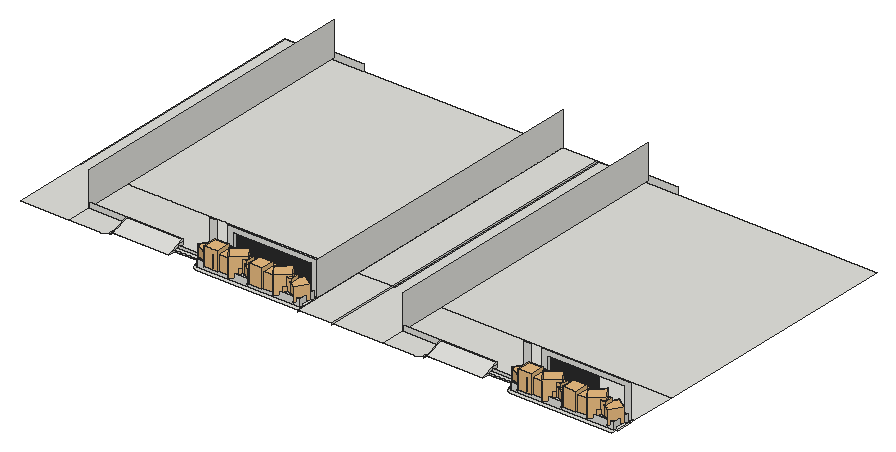
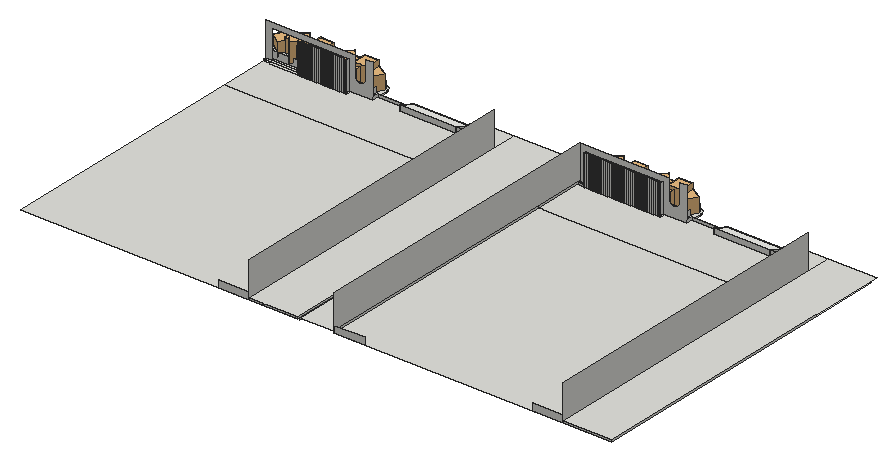
# SketchUp Ruby script. Lengths in inches.
U = 1.inch
M = Sketchup.active_model
def pt(a) = Geom::Point3d.new(a.map { |v| v * U })
def face(e, loops, mat)
  f = e.add_face(loops[0].map { |a| pt(a) })
  loops[1..].each { |l| e.add_face(l.map { |a| pt(a) }).erase! }
  f.material = f.back_material = mat if mat
  f
end
# faces: each face lists its corners as indices into pts; further lists are holes
def faces(e, pts, list, mat = nil) = list.each { |f| face(e, (f[0].is_a?(Array) ? f : [f]).map { |l| l.map { |i| pts[i] } }, mat) }
# xy, xz, yz: faces in a plane at the given z, y or x. An outline is a flat list of corners, or four numbers for a rectangle; further outlines are holes
def ring(l) = l.size == 4 ? [[l[0], l[1]], [l[2], l[1]], [l[2], l[3]], [l[0], l[3]]] : l.each_slice(2).to_a
def flat(e, list, mat, &to3) = list.each { |f| face(e, (f[0].is_a?(Array) ? f : [f]).map { |l| ring(l).map { |u, v| to3.(u, v) } }, mat) }
def xy(e, z, list, mat = nil) = flat(e, list, mat) { |x, y| [x, y, z] }
def xz(e, y, list, mat = nil) = flat(e, list, mat) { |x, z| [x, y, z] }
def yz(e, x, list, mat = nil) = flat(e, list, mat) { |y, z| [x, y, z] }
def lines(e, pts, list) = list.each { |a, b| e.add_line(pt(pts[a]), pt(pts[b])) }
# prism: a flat outline (further loops are holes) pulled along v
def prism(e, loops, v, mat = nil)
  f = face(e, loops, mat); d = Geom::Vector3d.new(v.map { |x| x * U })
  f.pushpull(f.normal.samedirection?(d) ? d.length : -d.length)
end
def box(e, o, s, mat = nil) = prism(e, [[o, [o[0] + s[0], o[1], o[2]], [o[0] + s[0], o[1] + s[1], o[2]], [o[0], o[1] + s[1], o[2]]]], [0, 0, s[2]], mat)
def at(x, y, z, deg = 0) = Geom::Transformation.translation(pt([x, y, z])) * Geom::Transformation.rotation(ORIGIN, Z_AXIS, deg.degrees)
def axes(o, x, y, z) = Geom::Transformation.new([*x, 0, *y, 0, *z, 0, *pt(o).to_a, 1])
def part(name) = M.definitions.add(name)
# library, detail: a bought-in or finely detailed component or shape, given as its bounding box
def library(name, o, s) = part(name).tap { |d| box(d.entities, o, s) }
def detail(e, o, s) = box(e.add_group.entities, o, s)
def put(e, d, t, mat = nil) = e.add_instance(d, t).tap { |i| i.material = mat if mat }
def group(e, t, mat = nil) = e.add_group.tap { |g| g.transformation = t; g.material = mat if mat }.entities
root = M.entities
M.materials.add("Material__1").color = [95, 70, 46]
M.materials.add("[0041_Chocolate]").color = [210, 105, 30]
c1 = library("Areca palm plant",[0,0,0],[49.1,36.6,54.46])
c2 = library("Group\#74",[-84.69,-90.07,-0.36],[176.51,175.13,171.4])
c3 = library("Group20\#1",[-20.81,-17.08,3.79],[39.86,39.43,37.51])
c4 = library("Group38\#2",[14.01,28.44,-23.43],[18.58,18.32,38.89])
c5 = library("Group\#130",[-7.34,-1.2,0],[38.67,35.81,49.04])
c6 = part("Group\#8")
put(c6.entities,c1,axes([-6.2,56.6,6.08],[0.45017,-0.56191,0],[0.66137,0.52986,0],[0,0,0.72]))
put(c6.entities,c1,axes([-6.2,158.41,6.08],[0.45017,-0.56191,0],[0.66137,0.52986,0],[0,0,0.72]))
put(c6.entities,c2,axes([14.93,145.87,6.05],[-0.04961,-0.08593,0],[0.08593,-0.04961,0],[0,0,0.10522]))
put(c6.entities,c2,axes([14.93,193.18,6.05],[-0.04961,-0.08593,0],[0.08593,-0.04961,0],[0,0,0.10522]))
put(c6.entities,c3,axes([18.97,79.98,4.77],[0,0.85,0],[-0.85,0,0],[0,0,0.85]))
put(c6.entities,c2,axes([14.93,173.12,6.05],[-0.04961,-0.08593,0],[0.08593,-0.04961,0],[0,0,0.10522]))
g1 = group(c6.entities,at(0,0,0))
xy(g1,0,[[0,0,6,234.8],[30,0,36,234.8]])
xy(g1,3,[[6,0,30,234.8]])
xy(g1,7,[[6,5,30,229.8]],"Material__1")
xy(g1,15,[[[0,0,36,234.8],[6,5,30,229.8]]])
xz(g1,0,[[0,0,6,0,6,3,30,3,30,0,36,0,36,15,0,15]])
xz(g1,5,[[6,7,30,15]])
xz(g1,229.8,[[6,7,30,15]])
xz(g1,234.8,[[0,0,0,15,36,15,36,0,30,0,30,3,6,3,6,0]])
yz(g1,0,[[0,0,234.8,15]])
yz(g1,6,[[0,0,234.8,3],[5,7,229.8,15]])
yz(g1,30,[[0,0,234.8,3],[5,7,229.8,15]])
yz(g1,36,[[0,0,234.8,15]])
put(c6.entities,c2,axes([17.19,223.04,6.07],[-0.08133,-0.14087,0],[0.14087,-0.08133,0],[0,0,0.1725]))
put(c6.entities,c4,axes([-4.1,-1.15,28.17],[0.8848,0,0],[0,0.94674,0],[0,0,0.85826]))
put(c6.entities,c2,axes([17.19,15.79,6.07],[-0.08133,-0.14087,0],[0.14087,-0.08133,0],[0,0,0.1725]))
put(c6.entities,c2,axes([14.93,91.37,6.05],[-0.04961,-0.08593,0],[0.08593,-0.04961,0],[0,0,0.10522]))
put(c6.entities,c3,axes([18.97,181.79,4.77],[0,0.85,0],[-0.85,0,0],[0,0,0.85]))
put(c6.entities,c2,axes([14.93,44.05,6.05],[-0.04961,-0.08593,0],[0.08593,-0.04961,0],[0,0,0.10522]))
put(c6.entities,c5,axes([24.9375,191.72,8],[0,0.79,0],[-0.79,0,0],[0,0,0.79]))
put(c6.entities,c2,axes([17.19,121.23,6.07],[-0.08133,-0.14087,0],[0.14087,-0.08133,0],[0,0,0.1725]))
put(c6.entities,c4,axes([-4.1,100.66,28.17],[0.8848,0,0],[0,0.94674,0],[0,0,0.85826]))
put(c6.entities,c5,axes([24.9375,89.91,8],[0,0.79,0],[-0.79,0,0],[0,0,0.79]))
put(c6.entities,c2,axes([14.93,71.3,6.05],[-0.04961,-0.08593,0],[0.08593,-0.04961,0],[0,0,0.10522]))
xy(root,-8,[[762.73,853.22,811.8125,853.22,811.8125,894.77,813.4375,894.77,813.4375,895.77,814.1875,895.77,814.1875,894.77,817.4375,894.77,817.4375,895.77,818.1875,895.77,818.1875,894.77,821.4375,894.77,821.4375,895.77,822.1875,895.77,822.1875,894.77,825.4375,894.77,825.4375,895.77,826.1875,895.77,826.1875,894.77,829.4375,894.77,829.4375,895.77,830.1875,895.77,830.1875,894.77,833.4375,894.77,833.4375,895.77,834.1875,895.77,834.1875,894.77,837.4375,894.77,837.4375,895.77,838.1875,895.77,838.1875,894.77,841.4375,894.77,841.4375,895.77,842.1875,895.77,842.1875,894.77,845.4375,894.77,845.4375,895.77,846.1875,895.77,846.1875,894.77,849.4375,894.77,849.4375,895.77,850.1875,895.77,850.1875,894.77,853.4375,894.77,853.4375,895.77,854.1875,895.77,854.1875,894.77,857.4375,894.77,857.4375,895.77,858.1875,895.77,858.1875,894.77,861.4375,894.77,861.4375,895.77,862.1875,895.77,862.1875,894.77,865.4375,894.77,865.4375,895.77,866.1875,895.77,866.1875,894.77,869.4375,894.77,869.4375,895.77,870.1875,895.77,870.1875,894.77,873.4375,894.77,873.4375,895.77,874.1875,895.77,874.1875,894.77,877.4375,894.77,877.4375,895.77,878.1875,895.77,878.1875,894.77,881.4375,894.77,881.4375,895.77,882.1875,895.77,882.1875,894.77,885.4375,894.77,885.4375,895.77,886.1875,895.77,886.1875,894.77,889.4375,894.77,889.4375,895.77,890.1875,895.77,890.1875,894.77,893.4375,894.77,893.4375,895.77,894.1875,895.77,894.1875,894.77,897.4375,894.77,897.4375,895.77,898.1875,895.77,898.1875,894.77,901.4375,894.77,901.4375,895.77,902.1875,895.77,902.1875,894.77,905.4375,894.77,905.4375,895.77,906.1875,895.77,906.1875,894.77,909.4375,894.77,909.4375,895.77,910.1875,895.77,910.1875,894.77,913.4375,894.77,913.4375,895.77,914.1875,895.77,914.1875,894.77,917.4375,894.77,917.4375,895.77,918.1875,895.77,918.1875,894.77,921.4375,894.77,921.4375,895.77,922.1875,895.77,922.1875,894.77,925.4375,894.77,925.4375,895.77,926.1875,895.77,926.1875,894.77,929.4375,894.77,929.4375,895.77,930.1875,895.77,930.1875,894.77,933.4375,894.77,933.4375,895.77,934.1875,895.77,934.1875,894.77,937.4375,894.77,937.4375,895.77,938.1875,895.77,938.1875,894.77,941.4375,894.77,941.4375,895.77,942.1875,895.77,942.1875,894.77,945.4375,894.77,945.4375,895.77,946.1875,895.77,946.1875,894.77,949.4375,894.77,949.4375,895.77,950.1875,895.77,950.1875,894.77,953.4375,894.77,953.4375,895.77,954.1875,895.77,954.1875,894.77,957.4375,894.77,957.4375,895.77,958.1875,895.77,958.1875,894.77,961.4375,894.77,961.4375,895.77,962.1875,895.77,962.1875,894.77,965.4375,894.77,965.4375,895.77,966.1875,895.77,966.1875,894.77,969.4375,894.77,969.4375,895.77,970.1875,895.77,970.1875,894.77,986.33,894.77,986.33,996.48,407.52,996.48,407.52,853.41,705.71,853.41,705.71,868.96,762.73,868.96],[811.8125,853.22,811.8125,894.77,973.4375,894.77,973.4375,889.52,986.33,889.52,986.33,853.22],[1418.23,853.22,1467.3125,853.22,1467.3125,894.77,1468.9375,894.77,1468.9375,895.77,1469.6875,895.77,1469.6875,894.77,1472.9375,894.77,1472.9375,895.77,1473.6875,895.77,1473.6875,894.77,1476.9375,894.77,1476.9375,895.77,1477.6875,895.77,1477.6875,894.77,1480.9375,894.77,1480.9375,895.77,1481.6875,895.77,1481.6875,894.77,1484.9375,894.77,1484.9375,895.77,1485.6875,895.77,1485.6875,894.77,1488.9375,894.77,1488.9375,895.77,1489.6875,895.77,1489.6875,894.77,1492.9375,894.77,1492.9375,895.77,1493.6875,895.77,1493.6875,894.77,1496.9375,894.77,1496.9375,895.77,1497.6875,895.77,1497.6875,894.77,1500.9375,894.77,1500.9375,895.77,1501.6875,895.77,1501.6875,894.77,1504.9375,894.77,1504.9375,895.77,1505.6875,895.77,1505.6875,894.77,1508.9375,894.77,1508.9375,895.77,1509.6875,895.77,1509.6875,894.77,1512.9375,894.77,1512.9375,895.77,1513.6875,895.77,1513.6875,894.77,1516.9375,894.77,1516.9375,895.77,1517.6875,895.77,1517.6875,894.77,1520.9375,894.77,1520.9375,895.77,1521.6875,895.77,1521.6875,894.77,1524.9375,894.77,1524.9375,895.77,1525.6875,895.77,1525.6875,894.77,1528.9375,894.77,1528.9375,895.77,1529.6875,895.77,1529.6875,894.77,1532.9375,894.77,1532.9375,895.77,1533.6875,895.77,1533.6875,894.77,1536.9375,894.77,1536.9375,895.77,1537.6875,895.77,1537.6875,894.77,1540.9375,894.77,1540.9375,895.77,1541.6875,895.77,1541.6875,894.77,1544.9375,894.77,1544.9375,895.77,1545.6875,895.77,1545.6875,894.77,1548.9375,894.77,1548.9375,895.77,1549.6875,895.77,1549.6875,894.77,1552.9375,894.77,1552.9375,895.77,1553.6875,895.77,1553.6875,894.77,1556.9375,894.77,1556.9375,895.77,1557.6875,895.77,1557.6875,894.77,1560.9375,894.77,1560.9375,895.77,1561.6875,895.77,1561.6875,894.77,1564.9375,894.77,1564.9375,895.77,1565.6875,895.77,1565.6875,894.77,1568.9375,894.77,1568.9375,895.77,1569.6875,895.77,1569.6875,894.77,1572.9375,894.77,1572.9375,895.77,1573.6875,895.77,1573.6875,894.77,1576.9375,894.77,1576.9375,895.77,1577.6875,895.77,1577.6875,894.77,1580.9375,894.77,1580.9375,895.77,1581.6875,895.77,1581.6875,894.77,1584.9375,894.77,1584.9375,895.77,1585.6875,895.77,1585.6875,894.77,1588.9375,894.77,1588.9375,895.77,1589.6875,895.77,1589.6875,894.77,1592.9375,894.77,1592.9375,895.77,1593.6875,895.77,1593.6875,894.77,1596.9375,894.77,1596.9375,895.77,1597.6875,895.77,1597.6875,894.77,1600.9375,894.77,1600.9375,895.77,1601.6875,895.77,1601.6875,894.77,1604.9375,894.77,1604.9375,895.77,1605.6875,895.77,1605.6875,894.77,1608.9375,894.77,1608.9375,895.77,1609.6875,895.77,1609.6875,894.77,1612.9375,894.77,1612.9375,895.77,1613.6875,895.77,1613.6875,894.77,1616.9375,894.77,1616.9375,895.77,1617.6875,895.77,1617.6875,894.77,1620.9375,894.77,1620.9375,895.77,1621.6875,895.77,1621.6875,894.77,1624.9375,894.77,1624.9375,895.77,1625.6875,895.77,1625.6875,894.77,1641.83,894.77,1641.83,996.48,1063.02,996.48,1063.02,853.41,1361.21,853.41,1361.21,868.96,1418.23,868.96],[1467.3125,853.22,1467.3125,894.77,1628.9375,894.77,1628.9375,889.52,1641.83,889.52,1641.83,853.22],[973.4375,889.52,986.33,894.77],
  [407.52,996.48,986.33,1529.04],[1063.02,996.48,1641.83,1529.04]])
xy(root,-4.67,[[407.52,838.14,508.71,1529.04],[508.71,838.14,573,838.14,575,838.27,576.96,838.66,578.85,839.31,580.64,840.19,582.3,841.3,583.8,842.62,585.12,844.12,586.23,845.78,587.11,847.57,587.75,849.46,588.14,851.42,588.27,853.41,588.27,889.52,508.71,889.52],[777.8125,838.14,986.33,838.14,986.33,889.52,762.73,889.52,762.73,853.22,762.86,851.26,763.24,849.32,763.88,847.45,764.75,845.68,765.85,844.04,767.15,842.5625,768.63,841.26,770.27,840.16,772.04,839.29,773.91,838.66,775.84,838.27],[986.33,838.14,1058.02,996.48],[1063.02,838.14,1164.21,1529.04],
  [1164.21,838.14,1228.5,838.14,1230.5,838.27,1232.46,838.66,1234.35,839.31,1236.14,840.19,1237.8,841.3,1239.3,842.62,1240.62,844.12,1241.73,845.78,1242.61,847.57,1243.25,849.46,1243.64,851.42,1243.77,853.41,1243.77,889.52,1164.21,889.52],[1433.3125,838.14,1641.83,838.14,1641.83,889.52,1418.23,889.52,1418.23,853.22,1418.36,851.26,1418.74,849.32,1419.38,847.45,1420.25,845.68,1421.35,844.04,1422.65,842.5625,1424.13,841.26,1425.77,840.16,1427.54,839.29,1429.41,838.66,1431.34,838.27],[705.71,868.96,762.73,876.83],[1361.21,868.96,1418.23,876.83],[811.8125,889.52,986.33,894.77],
  [1467.3125,889.52,1641.83,894.77],[986.33,996.48,1058.02,1529.04]])
xz(root,868.96,[[705.71,-8,762.73,-4.67],[1361.21,-8,1418.23,-4.67]])
xz(root,876.83,[[705.71,-4.67,762.73,0.73],[1361.21,-4.67,1418.23,0.73]])
xz(root,889.52,[[973.4375,-8,986.33,-4.67],[508.71,-4.67,588.27,6.125],[588.27,-4.67,705.71,6.125],[762.73,-4.67,811.8125,-4.67,811.8125,55.1875,973.4375,55.1875,973.4375,-4.67,986.33,-4.67,986.33,66.125,800.41,66.125,800.41,26.79,799.52,24.11,798.06,21.71,796.09,19.69,793.71,18.17,791.05,17.23,788.25,16.91,785.45,17.23,782.8,18.17,780.42,19.69,778.45,21.71,776.98,24.11,776.1,26.79,776.1,66.125,762.97,66.125,762.97,6.125,762.73,6.125],[1164.21,-4.67,1243.77,6.125],
  [1243.77,-4.67,1361.21,6.125],[1418.23,-4.67,1467.3125,-4.67,1467.3125,55.1875,1628.9375,55.1875,1628.9375,-4.67,1641.83,-4.67,1641.83,66.125,1455.91,66.125,1455.91,26.79,1455.02,24.11,1453.56,21.71,1451.59,19.69,1449.21,18.17,1446.55,17.23,1443.75,16.91,1440.95,17.23,1438.3,18.17,1435.92,19.69,1433.95,21.71,1432.48,24.11,1431.6,26.79,1431.6,66.125,1418.47,66.125,1418.47,6.125,1418.23,6.125]])
xz(root,894.77,[[811.8125,-8,813.4375,-4.67],[813.4375,-8,814.1875,-4.67],[814.1875,-8,817.4375,-4.67],[817.4375,-8,818.1875,-4.67],[818.1875,-8,821.4375,-4.67],
  [821.4375,-8,822.1875,-4.67],[822.1875,-8,825.4375,-4.67],[825.4375,-8,826.1875,-4.67],[826.1875,-8,829.4375,-4.67],[829.4375,-8,830.1875,-4.67],
  [830.1875,-8,833.4375,-4.67],[833.4375,-8,834.1875,-4.67],[834.1875,-8,837.4375,-4.67],[837.4375,-8,838.1875,-4.67],[838.1875,-8,841.4375,-4.67],
  [841.4375,-8,842.1875,-4.67],[842.1875,-8,845.4375,-4.67],[845.4375,-8,846.1875,-4.67],[846.1875,-8,849.4375,-4.67],[849.4375,-8,850.1875,-4.67],
  [850.1875,-8,853.4375,-4.67],[853.4375,-8,854.1875,-4.67],[854.1875,-8,857.4375,-4.67],[857.4375,-8,858.1875,-4.67],[858.1875,-8,861.4375,-4.67],
  [861.4375,-8,862.1875,-4.67],[862.1875,-8,865.4375,-4.67],[865.4375,-8,866.1875,-4.67],[866.1875,-8,869.4375,-4.67],[869.4375,-8,870.1875,-4.67],
  [870.1875,-8,873.4375,-4.67],[873.4375,-8,874.1875,-4.67],[874.1875,-8,877.4375,-4.67],[877.4375,-8,878.1875,-4.67],[878.1875,-8,881.4375,-4.67],
  [881.4375,-8,882.1875,-4.67],[882.1875,-8,885.4375,-4.67],[885.4375,-8,886.1875,-4.67],[886.1875,-8,889.4375,-4.67],[889.4375,-8,890.1875,-4.67],
  [890.1875,-8,893.4375,-4.67],[893.4375,-8,894.1875,-4.67],[894.1875,-8,897.4375,-4.67],[897.4375,-8,898.1875,-4.67],[898.1875,-8,901.4375,-4.67],
  [901.4375,-8,902.1875,-4.67],[902.1875,-8,905.4375,-4.67],[905.4375,-8,906.1875,-4.67],[906.1875,-8,909.4375,-4.67],[909.4375,-8,910.1875,-4.67],
  [910.1875,-8,913.4375,-4.67],[913.4375,-8,914.1875,-4.67],[914.1875,-8,917.4375,-4.67],[917.4375,-8,918.1875,-4.67],[918.1875,-8,921.4375,-4.67],
  [921.4375,-8,922.1875,-4.67],[922.1875,-8,925.4375,-4.67],[925.4375,-8,926.1875,-4.67],[926.1875,-8,929.4375,-4.67],[929.4375,-8,930.1875,-4.67],
  [930.1875,-8,933.4375,-4.67],[933.4375,-8,934.1875,-4.67],[934.1875,-8,937.4375,-4.67],[937.4375,-8,938.1875,-4.67],[938.1875,-8,941.4375,-4.67],
  [941.4375,-8,942.1875,-4.67],[942.1875,-8,945.4375,-4.67],[945.4375,-8,946.1875,-4.67],[946.1875,-8,949.4375,-4.67],[949.4375,-8,950.1875,-4.67],
  [950.1875,-8,953.4375,-4.67],[953.4375,-8,954.1875,-4.67],[954.1875,-8,957.4375,-4.67],[957.4375,-8,958.1875,-4.67],[958.1875,-8,961.4375,-4.67],
  [961.4375,-8,962.1875,-4.67],[962.1875,-8,965.4375,-4.67],[965.4375,-8,966.1875,-4.67],[966.1875,-8,969.4375,-4.67],[969.4375,-8,970.1875,-4.67],
  [970.1875,-8,973.4375,-4.67],[973.4375,-8,986.33,-4.67],[1467.3125,-8,1468.9375,-4.67],[1468.9375,-8,1469.6875,-4.67],[1469.6875,-8,1472.9375,-4.67],
  [1472.9375,-8,1473.6875,-4.67],[1473.6875,-8,1476.9375,-4.67],[1476.9375,-8,1477.6875,-4.67],[1477.6875,-8,1480.9375,-4.67],[1480.9375,-8,1481.6875,-4.67],
  [1481.6875,-8,1484.9375,-4.67],[1484.9375,-8,1485.6875,-4.67],[1485.6875,-8,1488.9375,-4.67],[1488.9375,-8,1489.6875,-4.67],[1489.6875,-8,1492.9375,-4.67],
  [1492.9375,-8,1493.6875,-4.67],[1493.6875,-8,1496.9375,-4.67],[1496.9375,-8,1497.6875,-4.67],[1497.6875,-8,1500.9375,-4.67],[1500.9375,-8,1501.6875,-4.67],
  [1501.6875,-8,1504.9375,-4.67],[1504.9375,-8,1505.6875,-4.67],[1505.6875,-8,1508.9375,-4.67],[1508.9375,-8,1509.6875,-4.67],[1509.6875,-8,1512.9375,-4.67],
  [1512.9375,-8,1513.6875,-4.67],[1513.6875,-8,1516.9375,-4.67],[1516.9375,-8,1517.6875,-4.67],[1517.6875,-8,1520.9375,-4.67],[1520.9375,-8,1521.6875,-4.67],
  [1521.6875,-8,1524.9375,-4.67],[1524.9375,-8,1525.6875,-4.67],[1525.6875,-8,1528.9375,-4.67],[1528.9375,-8,1529.6875,-4.67],[1529.6875,-8,1532.9375,-4.67],
  [1532.9375,-8,1533.6875,-4.67],[1533.6875,-8,1536.9375,-4.67],[1536.9375,-8,1537.6875,-4.67],[1537.6875,-8,1540.9375,-4.67],[1540.9375,-8,1541.6875,-4.67],
  [1541.6875,-8,1544.9375,-4.67],[1544.9375,-8,1545.6875,-4.67],[1545.6875,-8,1548.9375,-4.67],[1548.9375,-8,1549.6875,-4.67],[1549.6875,-8,1552.9375,-4.67],
  [1552.9375,-8,1553.6875,-4.67],[1553.6875,-8,1556.9375,-4.67],[1556.9375,-8,1557.6875,-4.67],[1557.6875,-8,1560.9375,-4.67],[1560.9375,-8,1561.6875,-4.67],
  [1561.6875,-8,1564.9375,-4.67],[1564.9375,-8,1565.6875,-4.67],[1565.6875,-8,1568.9375,-4.67],[1568.9375,-8,1569.6875,-4.67]])
xz(root,894.77,[[811.8125,-4.67,813.4375,55.1875],[814.1875,-4.67,817.4375,55.1875],[818.1875,-4.67,821.4375,55.1875],[822.1875,-4.67,825.4375,55.1875],[826.1875,-4.67,829.4375,55.1875],
  [830.1875,-4.67,833.4375,55.1875],[834.1875,-4.67,837.4375,55.1875],[838.1875,-4.67,841.4375,55.1875],[842.1875,-4.67,845.4375,55.1875],[846.1875,-4.67,849.4375,55.1875],
  [850.1875,-4.67,853.4375,55.1875],[854.1875,-4.67,857.4375,55.1875],[858.1875,-4.67,861.4375,55.1875],[862.1875,-4.67,865.4375,55.1875],[866.1875,-4.67,869.4375,55.1875],
  [870.1875,-4.67,873.4375,55.1875],[874.1875,-4.67,877.4375,55.1875],[878.1875,-4.67,881.4375,55.1875],[882.1875,-4.67,885.4375,55.1875],[886.1875,-4.67,889.4375,55.1875],
  [890.1875,-4.67,893.4375,55.1875],[894.1875,-4.67,897.4375,55.1875],[898.1875,-4.67,901.4375,55.1875],[902.1875,-4.67,905.4375,55.1875],[906.1875,-4.67,909.4375,55.1875],
  [910.1875,-4.67,913.4375,55.1875],[914.1875,-4.67,917.4375,55.1875],[918.1875,-4.67,921.4375,55.1875],[922.1875,-4.67,925.4375,55.1875],[926.1875,-4.67,929.4375,55.1875],
  [930.1875,-4.67,933.4375,55.1875],[934.1875,-4.67,937.4375,55.1875],[938.1875,-4.67,941.4375,55.1875],[942.1875,-4.67,945.4375,55.1875],[946.1875,-4.67,949.4375,55.1875],
  [950.1875,-4.67,953.4375,55.1875],[954.1875,-4.67,957.4375,55.1875],[958.1875,-4.67,961.4375,55.1875],[962.1875,-4.67,965.4375,55.1875],[966.1875,-4.67,969.4375,55.1875],
  [970.1875,-4.67,973.4375,55.1875],[1467.3125,-4.67,1468.9375,55.1875],[1469.6875,-4.67,1472.9375,55.1875],[1473.6875,-4.67,1476.9375,55.1875],[1477.6875,-4.67,1480.9375,55.1875],
  [1481.6875,-4.67,1484.9375,55.1875],[1485.6875,-4.67,1488.9375,55.1875],[1489.6875,-4.67,1492.9375,55.1875],[1493.6875,-4.67,1496.9375,55.1875],[1497.6875,-4.67,1500.9375,55.1875],
  [1501.6875,-4.67,1504.9375,55.1875],[1505.6875,-4.67,1508.9375,55.1875],[1509.6875,-4.67,1512.9375,55.1875],[1513.6875,-4.67,1516.9375,55.1875],[1517.6875,-4.67,1520.9375,55.1875],
  [1521.6875,-4.67,1524.9375,55.1875],[1525.6875,-4.67,1528.9375,55.1875],[1529.6875,-4.67,1532.9375,55.1875],[1533.6875,-4.67,1536.9375,55.1875],[1537.6875,-4.67,1540.9375,55.1875],
  [1541.6875,-4.67,1544.9375,55.1875],[1545.6875,-4.67,1548.9375,55.1875],[1549.6875,-4.67,1552.9375,55.1875],[1553.6875,-4.67,1556.9375,55.1875],[1557.6875,-4.67,1560.9375,55.1875],
  [1561.6875,-4.67,1564.9375,55.1875],[1565.6875,-4.67,1568.9375,55.1875]],"[0041_Chocolate]")
xz(root,895.77,[[813.4375,-8,814.1875,55.1875],[817.4375,-8,818.1875,55.1875],[821.4375,-8,822.1875,55.1875],[825.4375,-8,826.1875,55.1875],[829.4375,-8,830.1875,55.1875],
  [833.4375,-8,834.1875,55.1875],[837.4375,-8,838.1875,55.1875],[841.4375,-8,842.1875,55.1875],[845.4375,-8,846.1875,55.1875],[849.4375,-8,850.1875,55.1875],
  [853.4375,-8,854.1875,55.1875],[857.4375,-8,858.1875,55.1875],[861.4375,-8,862.1875,55.1875],[865.4375,-8,866.1875,55.1875],[869.4375,-8,870.1875,55.1875],
  [873.4375,-8,874.1875,55.1875],[877.4375,-8,878.1875,55.1875],[881.4375,-8,882.1875,55.1875],[885.4375,-8,886.1875,55.1875],[889.4375,-8,890.1875,55.1875],
  [893.4375,-8,894.1875,55.1875],[897.4375,-8,898.1875,55.1875],[901.4375,-8,902.1875,55.1875],[905.4375,-8,906.1875,55.1875],[909.4375,-8,910.1875,55.1875],
  [913.4375,-8,914.1875,55.1875],[917.4375,-8,918.1875,55.1875],[921.4375,-8,922.1875,55.1875],[925.4375,-8,926.1875,55.1875],[929.4375,-8,930.1875,55.1875],
  [933.4375,-8,934.1875,55.1875],[937.4375,-8,938.1875,55.1875],[941.4375,-8,942.1875,55.1875],[945.4375,-8,946.1875,55.1875],[949.4375,-8,950.1875,55.1875],
  [953.4375,-8,954.1875,55.1875],[957.4375,-8,958.1875,55.1875],[961.4375,-8,962.1875,55.1875],[965.4375,-8,966.1875,55.1875],[969.4375,-8,970.1875,55.1875],
  [1468.9375,-8,1469.6875,55.1875],[1472.9375,-8,1473.6875,55.1875],[1476.9375,-8,1477.6875,55.1875],[1480.9375,-8,1481.6875,55.1875],[1484.9375,-8,1485.6875,55.1875],
  [1488.9375,-8,1489.6875,55.1875],[1492.9375,-8,1493.6875,55.1875],[1496.9375,-8,1497.6875,55.1875],[1500.9375,-8,1501.6875,55.1875],[1504.9375,-8,1505.6875,55.1875],
  [1508.9375,-8,1509.6875,55.1875],[1512.9375,-8,1513.6875,55.1875],[1516.9375,-8,1517.6875,55.1875],[1520.9375,-8,1521.6875,55.1875],[1524.9375,-8,1525.6875,55.1875],
  [1528.9375,-8,1529.6875,55.1875],[1532.9375,-8,1533.6875,55.1875],[1536.9375,-8,1537.6875,55.1875],[1540.9375,-8,1541.6875,55.1875],[1544.9375,-8,1545.6875,55.1875],
  [1548.9375,-8,1549.6875,55.1875],[1552.9375,-8,1553.6875,55.1875],[1556.9375,-8,1557.6875,55.1875],[1560.9375,-8,1561.6875,55.1875],[1564.9375,-8,1565.6875,55.1875],
  [1568.9375,-8,1569.6875,55.1875]])
xz(root,1529.04,[[407.52,-8,407.52,-4.67,508.71,-4.67,508.71,6.125,572.21,6.125,572.21,-8],[922.83,-8,986.33,6.125],[1063.02,-8,1063.02,-4.67,1164.21,-4.67,1164.21,6.125,1227.71,6.125,1227.71,-8]])
yz(root,407.52,[[996.48,-8,1529.04,-4.67]])
yz(root,508.71,[[889.52,-4.67,1529.04,66.125]])
yz(root,588.27,[[853.41,-8,861.93,-4.67,853.41,-4.67],[861.93,-4.67,889.52,6.125,889.52,-4.67]])
yz(root,705.71,[[853.41,-8,868.96,-8,868.96,-4.67,861.93,-4.67],[861.93,-4.67,876.83,-4.67,876.83,0.73,889.52,0.73,889.52,6.125],[876.83,-4.67,889.52,0.73]])
yz(root,762.73,[[853.22,-8,868.96,-4.67],[876.83,-4.67,889.52,0.73]])
yz(root,811.8125,[[889.52,-4.67,894.77,55.1875]])
yz(root,813.4375,[[894.77,-8,895.77,55.1875]])
yz(root,814.1875,[[894.77,-8,895.77,55.1875]])
yz(root,817.4375,[[894.77,-8,895.77,55.1875]])
yz(root,818.1875,[[894.77,-8,895.77,55.1875]])
yz(root,821.4375,[[894.77,-8,895.77,55.1875]])
yz(root,822.1875,[[894.77,-8,895.77,55.1875]])
yz(root,825.4375,[[894.77,-8,895.77,55.1875]])
yz(root,826.1875,[[894.77,-8,895.77,55.1875]])
yz(root,829.4375,[[894.77,-8,895.77,55.1875]])
yz(root,830.1875,[[894.77,-8,895.77,55.1875]])
yz(root,833.4375,[[894.77,-8,895.77,55.1875]])
yz(root,834.1875,[[894.77,-8,895.77,55.1875]])
yz(root,837.4375,[[894.77,-8,895.77,55.1875]])
yz(root,838.1875,[[894.77,-8,895.77,55.1875]])
yz(root,841.4375,[[894.77,-8,895.77,55.1875]])
yz(root,842.1875,[[894.77,-8,895.77,55.1875]])
yz(root,845.4375,[[894.77,-8,895.77,55.1875]])
yz(root,846.1875,[[894.77,-8,895.77,55.1875]])
yz(root,849.4375,[[894.77,-8,895.77,55.1875]])
yz(root,850.1875,[[894.77,-8,895.77,55.1875]])
yz(root,853.4375,[[894.77,-8,895.77,55.1875]])
yz(root,854.1875,[[894.77,-8,895.77,55.1875]])
yz(root,857.4375,[[894.77,-8,895.77,55.1875]])
yz(root,858.1875,[[894.77,-8,895.77,55.1875]])
yz(root,861.4375,[[894.77,-8,895.77,55.1875]])
yz(root,862.1875,[[894.77,-8,895.77,55.1875]])
yz(root,865.4375,[[894.77,-8,895.77,55.1875]])
yz(root,866.1875,[[894.77,-8,895.77,55.1875]])
yz(root,869.4375,[[894.77,-8,895.77,55.1875]])
yz(root,870.1875,[[894.77,-8,895.77,55.1875]])
yz(root,873.4375,[[894.77,-8,895.77,55.1875]])
yz(root,874.1875,[[894.77,-8,895.77,55.1875]])
yz(root,877.4375,[[894.77,-8,895.77,55.1875]])
yz(root,878.1875,[[894.77,-8,895.77,55.1875]])
yz(root,881.4375,[[894.77,-8,895.77,55.1875]])
yz(root,882.1875,[[894.77,-8,895.77,55.1875]])
yz(root,885.4375,[[894.77,-8,895.77,55.1875]])
yz(root,886.1875,[[894.77,-8,895.77,55.1875]])
yz(root,889.4375,[[894.77,-8,895.77,55.1875]])
yz(root,890.1875,[[894.77,-8,895.77,55.1875]])
yz(root,893.4375,[[894.77,-8,895.77,55.1875]])
yz(root,894.1875,[[894.77,-8,895.77,55.1875]])
yz(root,897.4375,[[894.77,-8,895.77,55.1875]])
yz(root,898.1875,[[894.77,-8,895.77,55.1875]])
yz(root,901.4375,[[894.77,-8,895.77,55.1875]])
yz(root,902.1875,[[894.77,-8,895.77,55.1875]])
yz(root,905.4375,[[894.77,-8,895.77,55.1875]])
yz(root,906.1875,[[894.77,-8,895.77,55.1875]])
yz(root,909.4375,[[894.77,-8,895.77,55.1875]])
yz(root,910.1875,[[894.77,-8,895.77,55.1875]])
yz(root,913.4375,[[894.77,-8,895.77,55.1875]])
yz(root,914.1875,[[894.77,-8,895.77,55.1875]])
yz(root,917.4375,[[894.77,-8,895.77,55.1875]])
yz(root,918.1875,[[894.77,-8,895.77,55.1875]])
yz(root,921.4375,[[894.77,-8,895.77,55.1875]])
yz(root,922.1875,[[894.77,-8,895.77,55.1875]])
yz(root,925.4375,[[894.77,-8,895.77,55.1875]])
yz(root,926.1875,[[894.77,-8,895.77,55.1875]])
yz(root,929.4375,[[894.77,-8,895.77,55.1875]])
yz(root,930.1875,[[894.77,-8,895.77,55.1875]])
yz(root,933.4375,[[894.77,-8,895.77,55.1875]])
yz(root,934.1875,[[894.77,-8,895.77,55.1875]])
yz(root,937.4375,[[894.77,-8,895.77,55.1875]])
yz(root,938.1875,[[894.77,-8,895.77,55.1875]])
yz(root,941.4375,[[894.77,-8,895.77,55.1875]])
yz(root,942.1875,[[894.77,-8,895.77,55.1875]])
yz(root,945.4375,[[894.77,-8,895.77,55.1875]])
yz(root,946.1875,[[894.77,-8,895.77,55.1875]])
yz(root,949.4375,[[894.77,-8,895.77,55.1875]])
yz(root,950.1875,[[894.77,-8,895.77,55.1875]])
yz(root,953.4375,[[894.77,-8,895.77,55.1875]])
yz(root,954.1875,[[894.77,-8,895.77,55.1875]])
yz(root,957.4375,[[894.77,-8,895.77,55.1875]])
yz(root,958.1875,[[894.77,-8,895.77,55.1875]])
yz(root,961.4375,[[894.77,-8,895.77,55.1875]])
yz(root,962.1875,[[894.77,-8,895.77,55.1875]])
yz(root,965.4375,[[894.77,-8,895.77,55.1875]])
yz(root,966.1875,[[894.77,-8,895.77,55.1875]])
yz(root,969.4375,[[894.77,-8,895.77,55.1875]])
yz(root,970.1875,[[894.77,-8,895.77,55.1875]])
yz(root,973.4375,[[889.52,-8,894.77,55.1875]])
yz(root,986.33,[[838.14,-8,889.52,-4.67],[889.52,-8,894.77,-4.67],[894.77,-8,996.48,-4.67],[996.48,-8,1529.04,-4.67],[889.52,-4.67,1529.04,66.125]])
yz(root,1058.02,[[838.14,-8,996.48,-4.67],[996.48,-8,1529.04,-4.67]])
yz(root,1063.02,[[996.48,-8,1529.04,-4.67]])
yz(root,1164.21,[[889.52,-4.67,1529.04,66.125]])
yz(root,1243.77,[[853.41,-8,861.93,-4.67,853.41,-4.67],[861.93,-4.67,889.52,6.125,889.52,-4.67]])
yz(root,1361.21,[[853.41,-8,868.96,-8,868.96,-4.67,861.93,-4.67],[861.93,-4.67,876.83,-4.67,876.83,0.73,889.52,0.73,889.52,6.125],[876.83,-4.67,889.52,0.73]])
yz(root,1418.23,[[853.22,-8,868.96,-4.67],[876.83,-4.67,889.52,0.73]])
yz(root,1467.3125,[[889.52,-4.67,894.77,55.1875]])
yz(root,1468.9375,[[894.77,-8,895.77,55.1875]])
yz(root,1469.6875,[[894.77,-8,895.77,55.1875]])
yz(root,1472.9375,[[894.77,-8,895.77,55.1875]])
yz(root,1473.6875,[[894.77,-8,895.77,55.1875]])
yz(root,1476.9375,[[894.77,-8,895.77,55.1875]])
yz(root,1477.6875,[[894.77,-8,895.77,55.1875]])
yz(root,1480.9375,[[894.77,-8,895.77,55.1875]])
yz(root,1481.6875,[[894.77,-8,895.77,55.1875]])
yz(root,1484.9375,[[894.77,-8,895.77,55.1875]])
yz(root,1485.6875,[[894.77,-8,895.77,55.1875]])
yz(root,1488.9375,[[894.77,-8,895.77,55.1875]])
yz(root,1489.6875,[[894.77,-8,895.77,55.1875]])
yz(root,1492.9375,[[894.77,-8,895.77,55.1875]])
yz(root,1493.6875,[[894.77,-8,895.77,55.1875]])
yz(root,1496.9375,[[894.77,-8,895.77,55.1875]])
yz(root,1497.6875,[[894.77,-8,895.77,55.1875]])
yz(root,1500.9375,[[894.77,-8,895.77,55.1875]])
yz(root,1501.6875,[[894.77,-8,895.77,55.1875]])
yz(root,1504.9375,[[894.77,-8,895.77,55.1875]])
yz(root,1505.6875,[[894.77,-8,895.77,55.1875]])
yz(root,1508.9375,[[894.77,-8,895.77,55.1875]])
yz(root,1509.6875,[[894.77,-8,895.77,55.1875]])
yz(root,1512.9375,[[894.77,-8,895.77,55.1875]])
yz(root,1513.6875,[[894.77,-8,895.77,55.1875]])
yz(root,1516.9375,[[894.77,-8,895.77,55.1875]])
yz(root,1517.6875,[[894.77,-8,895.77,55.1875]])
yz(root,1520.9375,[[894.77,-8,895.77,55.1875]])
yz(root,1521.6875,[[894.77,-8,895.77,55.1875]])
yz(root,1524.9375,[[894.77,-8,895.77,55.1875]])
yz(root,1525.6875,[[894.77,-8,895.77,55.1875]])
yz(root,1528.9375,[[894.77,-8,895.77,55.1875]])
yz(root,1529.6875,[[894.77,-8,895.77,55.1875]])
yz(root,1532.9375,[[894.77,-8,895.77,55.1875]])
yz(root,1533.6875,[[894.77,-8,895.77,55.1875]])
yz(root,1536.9375,[[894.77,-8,895.77,55.1875]])
yz(root,1537.6875,[[894.77,-8,895.77,55.1875]])
yz(root,1540.9375,[[894.77,-8,895.77,55.1875]])
yz(root,1541.6875,[[894.77,-8,895.77,55.1875]])
yz(root,1544.9375,[[894.77,-8,895.77,55.1875]])
yz(root,1545.6875,[[894.77,-8,895.77,55.1875]])
yz(root,1548.9375,[[894.77,-8,895.77,55.1875]])
yz(root,1549.6875,[[894.77,-8,895.77,55.1875]])
yz(root,1552.9375,[[894.77,-8,895.77,55.1875]])
yz(root,1553.6875,[[894.77,-8,895.77,55.1875]])
yz(root,1556.9375,[[894.77,-8,895.77,55.1875]])
yz(root,1557.6875,[[894.77,-8,895.77,55.1875]])
yz(root,1560.9375,[[894.77,-8,895.77,55.1875]])
yz(root,1561.6875,[[894.77,-8,895.77,55.1875]])
yz(root,1564.9375,[[894.77,-8,895.77,55.1875]])
yz(root,1565.6875,[[894.77,-8,895.77,55.1875]])
yz(root,1568.9375,[[894.77,-8,895.77,55.1875]])
yz(root,1569.6875,[[894.77,-8,895.77,55.1875]])
p = [[1419.38,847.45,-4.67],[1418.74,849.32,-4.67],[1418.74,849.32,-8],[1419.38,847.45,-8],[587.75,849.46,-4.67],[587.11,847.57,-4.67],
  [587.11,847.57,-8],[587.75,849.46,-8],[1243.25,849.46,-4.67],[1242.61,847.57,-4.67],[1242.61,847.57,-8],[1243.25,849.46,-8],
  [763.24,849.32,-4.67],[762.86,851.26,-4.67],[762.86,851.26,-8],[763.24,849.32,-8],[1418.36,851.26,-4.67],[1418.36,851.26,-8],
  [588.14,851.42,-4.67],[588.14,851.42,-8],[1243.64,851.42,-4.67],[1243.64,851.42,-8],[762.73,853.22,-4.67],[762.73,853.22,-8],
  [1418.23,853.22,-4.67],[1418.23,853.22,-8],[588.27,853.41,-4.67],[588.27,853.41,-8],[1243.77,853.41,-4.67],[1243.77,853.41,-8],
  [705.71,853.41,-8],[705.71,861.93,-4.67],[705.71,889.52,6.125],[588.27,889.52,6.125],[588.27,861.93,-4.67],[1361.21,853.41,-8],
  [1361.21,861.93,-4.67],[1361.21,889.52,6.125],[1243.77,889.52,6.125],[1243.77,861.93,-4.67]]
faces(root,p,[[0,1,2,3],[4,5,6,7],[8,9,10,11],[12,13,14,15],[1,16,17,2],[18,4,7,19],[20,8,11,21],[13,22,23,14],
  [16,24,25,17],[26,18,19,27],[28,20,21,29],[30,31,32,33,34,27],[35,36,37,38,39,29]])
put(root,c6,axes([983.88,847.2,-4.73],[0,1,0],[-0.9127,0,0],[0,0,1]))
put(root,c6,axes([1639.38,847.2,-4.73],[0,1,0],[-0.9127,0,0],[0,0,1]))
